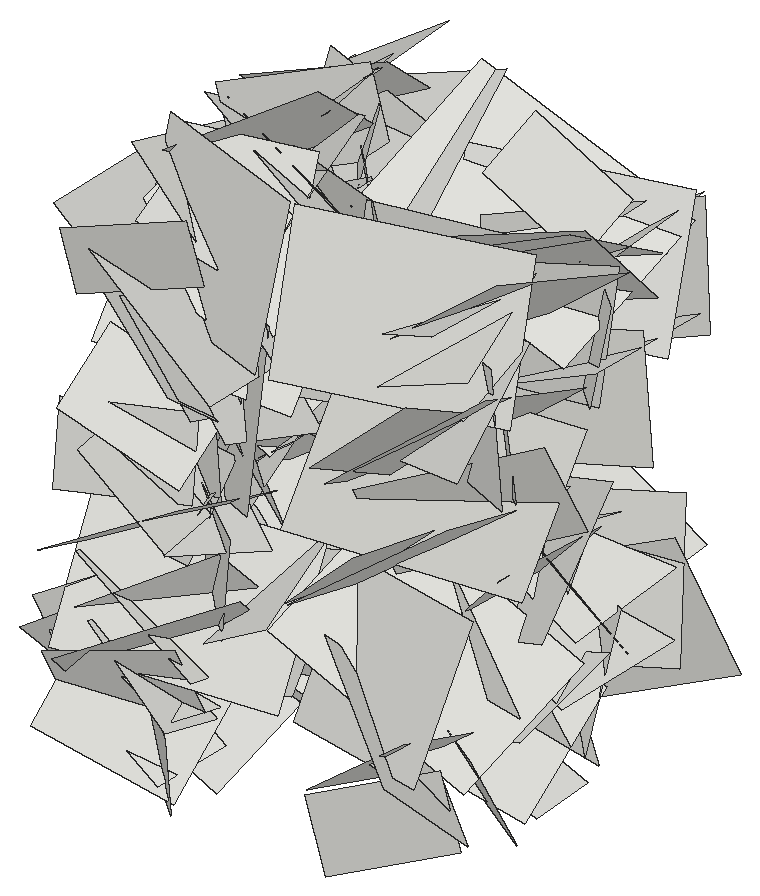
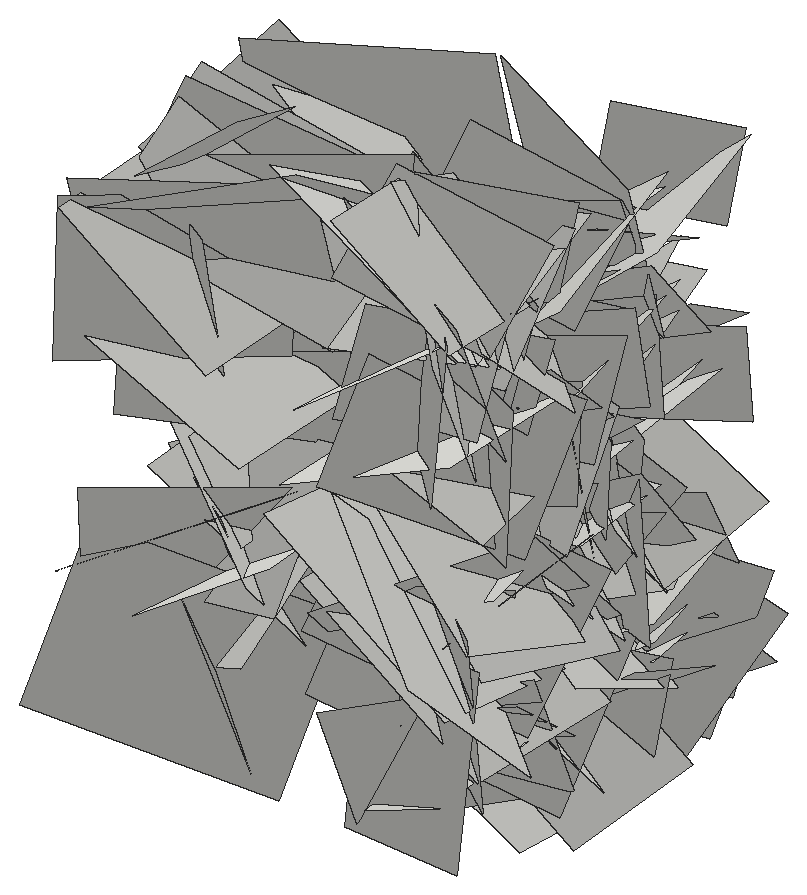
# SketchUp Ruby script. Lengths in inches.
U = 1.inch
M = Sketchup.active_model
def pt(a) = Geom::Point3d.new(a.map { |v| v * U })
def face(e, loops, mat)
  f = e.add_face(loops[0].map { |a| pt(a) })
  loops[1..].each { |l| e.add_face(l.map { |a| pt(a) }).erase! }
  f.material = f.back_material = mat if mat
  f
end
# faces: each face lists its corners as indices into pts; further lists are holes
def faces(e, pts, list, mat = nil) = list.each { |f| face(e, (f[0].is_a?(Array) ? f : [f]).map { |l| l.map { |i| pts[i] } }, mat) }
# xy, xz, yz: faces in a plane at the given z, y or x. An outline is a flat list of corners, or four numbers for a rectangle; further outlines are holes
def ring(l) = l.size == 4 ? [[l[0], l[1]], [l[2], l[1]], [l[2], l[3]], [l[0], l[3]]] : l.each_slice(2).to_a
def flat(e, list, mat, &to3) = list.each { |f| face(e, (f[0].is_a?(Array) ? f : [f]).map { |l| ring(l).map { |u, v| to3.(u, v) } }, mat) }
def xy(e, z, list, mat = nil) = flat(e, list, mat) { |x, y| [x, y, z] }
def xz(e, y, list, mat = nil) = flat(e, list, mat) { |x, z| [x, y, z] }
def yz(e, x, list, mat = nil) = flat(e, list, mat) { |y, z| [x, y, z] }
def lines(e, pts, list) = list.each { |a, b| e.add_line(pt(pts[a]), pt(pts[b])) }
# prism: a flat outline (further loops are holes) pulled along v
def prism(e, loops, v, mat = nil)
  f = face(e, loops, mat); d = Geom::Vector3d.new(v.map { |x| x * U })
  f.pushpull(f.normal.samedirection?(d) ? d.length : -d.length)
end
def box(e, o, s, mat = nil) = prism(e, [[o, [o[0] + s[0], o[1], o[2]], [o[0] + s[0], o[1] + s[1], o[2]], [o[0], o[1] + s[1], o[2]]]], [0, 0, s[2]], mat)
def at(x, y, z, deg = 0) = Geom::Transformation.translation(pt([x, y, z])) * Geom::Transformation.rotation(ORIGIN, Z_AXIS, deg.degrees)
def axes(o, x, y, z) = Geom::Transformation.new([*x, 0, *y, 0, *z, 0, *pt(o).to_a, 1])
def part(name) = M.definitions.add(name)
# library, detail: a bought-in or finely detailed component or shape, given as its bounding box
def library(name, o, s) = part(name).tap { |d| box(d.entities, o, s) }
def detail(e, o, s) = box(e.add_group.entities, o, s)
def put(e, d, t, mat = nil) = e.add_instance(d, t).tap { |i| i.material = mat if mat }
def group(e, t, mat = nil) = e.add_group.tap { |g| g.transformation = t; g.material = mat if mat }.entities
root = M.entities
c1 = part("Component\#6")
p = [[0.01,0,0],[0,3.24,4.54],[4.32,3.24,4.54],[4.33,0,0]]
faces(c1.entities,p,[[0,1,2,3]])
put(root,c1,axes([414.68,175.72,36.8],[0.15665,0.75943,0.7145],[0.11122,0.70715,-0.77331],[-1.09966,0.17971,0.02357]))
put(root,c1,axes([410.71,182.09,31.375],[0.0562,-0.72005,0.10613],[0.07977,0.11126,0.71729],[0.76737,0.04117,-0.08234]))
put(root,c1,axes([414.68,170.91,25.11],[-0.00896,0.33986,-0.6335],[-0.15678,-0.62081,-0.33108],[-0.74574,0.12644,0.07722]))
put(root,c1,axes([414.68,181.67,36.78],[0.05967,0.56874,-0.94691],[0.29528,-0.9248,-0.5389],[-1.13301,-0.21107,-0.19031]))
put(root,c1,axes([414.68,180.66,33.34],[0.08177,-0.45253,0.73357],[-0.03972,0.73405,0.45677],[-0.91278,-0.07248,0.04584]))
put(root,c1,axes([410.71,176.52,27.27],[0.06139,-0.83333,-0.30669],[-0.14477,-0.31205,0.82208],[0.93005,0.00643,0.1482]))
put(root,c1,axes([410.71,174.67,32.54],[-0.17055,0.3665,0.95024],[-0.03456,0.95968,-0.37566],[1.07902,0.08867,0.13816]))
put(root,c1,axes([410.71,177.99,23.55],[0.04107,0.5427,0.4395],[0.20397,0.41484,-0.52921],[0.71159,-0.15024,0.12632]))
put(root,c1,axes([410.71,177.89,30.77],[0.05678,-0.11721,0.8526],[-0.09083,0.84928,0.12214],[0.90772,0.09231,-0.04111]))
put(root,c1,axes([410.71,174.875,32.24],[0.12053,0.70886,0.38052],[-0.08644,0.39248,-0.70676],[0.84842,-0.06072,-0.12606]))
put(root,c1,axes([410.71,176.26,32.94],[0.03084,0.60524,0.59943],[-0.03406,0.60013,-0.60439],[0.90231,0.00196,-0.0433]))
put(root,c1,axes([410.71,169.05,21.98],[0.04882,0.58162,0.59704],[-0.02934,0.59868,-0.58109],[0.88303,-0.01226,-0.05232]))
put(root,c1,axes([410.71,171.18,26.98],[-0.09963,0.88743,-0.23237],[0.05305,-0.22828,-0.89204],[0.97094,0.10354,0.02489]))
put(root,c1,axes([410.71,174.16,29.86],[0.19319,0.59277,-0.26834],[0.07097,-0.29428,-0.60458],[0.68606,-0.13648,0.1381]))
put(root,c1,axes([414.68,171.52,27.71],[0.03995,0.48298,0.66079],[0.01207,0.66111,-0.48387],[-0.8675,0.03144,0.0237]))
put(root,c1,axes([410.71,174.95,31.63],[0.12097,-0.07785,-0.70642],[0.09105,-0.70871,0.09198],[0.74781,0.09888,0.10307]))
put(root,c1,axes([410.71,178.01,36.42],[0.04909,-0.68925,0.58112],[-0.09024,0.57594,0.68989],[0.95135,0.0902,0.03545]))
put(root,c1,axes([410.71,172,20.82],[-0.19013,-0.4174,1.11707],[-0.18593,1.12659,0.39279],[1.25031,0.10406,0.22828]))
put(root,c1,axes([414.68,172.01,32.68],[-0.01531,-0.04852,-0.71126],[-0.05574,-0.70939,0.04946],[-0.75363,0.05345,0.01079]))
put(root,c1,axes([410.71,184.3,37.98],[-0.01849,-0.42221,-1.00939],[-0.24573,-0.98518,0.41609],[1.13346,-0.22047,0.07374]))
put(root,c1,axes([410.71,183.5625,38.07],[0.03427,-0.86867,-0.02883],[-0.01016,-0.0292,0.8692],[0.92124,0.03199,0.01066]))
put(root,c1,axes([410.71,175.14,30.45],[-0.22771,0.17317,-1.07869],[0.0194,-1.09862,-0.18001],[1.15789,0.05246,-0.20912]))
put(root,c1,axes([414.68,173.36,27.66],[0.12062,0.63946,0.63128],[0.06443,0.62939,-0.6485],[-0.9503,0.12384,0.03616]))
put(root,c1,axes([414.68,173.29,20.87],[-0.09428,-0.62013,-0.08152],[-0.03551,-0.0775,0.6261],[-0.66205,0.09247,-0.02197]))
put(root,c1,axes([410.71,180.04,24.28],[0.15161,0.71603,-0.23582],[0.04269,-0.24694,-0.72538],[0.79796,-0.12284,0.08362]))
put(root,c1,axes([410.71,178.05,19.9375],[-0.14578,-1.0409,0.22357],[-0.02192,0.228,1.04879],[1.1283,-0.13006,0.04926]))
put(root,c1,axes([410.71,171.36,22.89],[0.02535,0.88672,0.32576],[-0.06435,0.32663,-0.88464],[0.99927,-0.00146,-0.06523]))
put(root,c1,axes([410.71,176.41,32.2],[0.11408,-0.0942,-0.79779],[0.0272,-0.8041,0.09841],[0.85109,0.03832,0.10379]))
put(root,c1,axes([414.68,177.7,39.03],[0.08239,-0.33737,-0.64844],[-0.10668,-0.65083,0.32654],[-0.76743,0.05425,-0.11501]))
put(root,c1,axes([410.71,181.8125,37.17],[-0.0246,-0.63961,0.56311],[0.17949,0.54862,0.63013],[0.88529,-0.129,-0.11211]))
put(root,c1,axes([410.71,173.5,20.5],[-0.29119,-0.77592,0.90535],[0.00734,0.92801,0.79744],[1.26387,-0.18415,0.20396]))
put(root,c1,axes([410.71,172.625,27.43],[-0.01975,0.58315,0.74345],[0.01761,0.74368,-0.58292],[1.00141,-0.00157,0.02491]))
put(root,c1,axes([410.71,172.13,35.78],[0.07615,0.65901,-0.5201],[0.04859,-0.52431,-0.658],[0.88857,-0.02781,0.08055]))
put(root,c1,axes([410.71,177.13,31.79],[-0.078,-0.30439,1.03044],[-0.07955,1.03178,0.29943],[1.13614,0.05135,0.09171]))
put(root,c1,axes([410.71,182.1,27.04],[-0.18817,-1.1788,-0.21223],[-0.10509,-0.19936,1.19019],[1.26526,-0.19187,0.06729]))
put(root,c1,axes([414.68,180.11,41],[0.0874,0.13713,-0.78202],[0.02965,-0.78624,-0.13492],[-0.84107,-0.01347,-0.08602]))
put(root,c1,axes([414.68,171.42,39.46],[-0.01769,0.21401,-0.61924],[-0.03571,-0.6189,-0.21298],[-0.69357,0.02641,0.02676]))
put(root,c1,axes([414.68,174.375,32.02],[0.18574,0.64681,-0.5499],[0.00393,-0.56207,-0.65994],[-0.8999,0.13105,-0.11638]))
put(root,c1,axes([414.68,173.15,22.23],[-0.01199,-0.5915,0.12784],[-0.10227,0.12799,0.58366],[-0.63327,-0.00947,-0.09668]))
put(root,c1,axes([410.71,170.16,39.2],[-0.24703,1.2789,-0.21613],[-0.13589,-0.24123,-1.28918],[1.36812,0.20696,-0.16707]))
put(root,c1,axes([410.71,174.01,26.46],[-0.07872,-0.97306,0.24072],[0.0738,0.23579,0.97461],[1.05998,-0.08868,-0.04998]))
put(root,c1,axes([414.68,173.67,32.24],[0.05341,-0.65994,-0.37026],[0.06447,-0.36634,0.66124],[-0.79951,-0.07362,0.02859]))
put(root,c1,axes([414.68,175.43,34.87],[0.0411,0.62613,0.35799],[0.03637,0.3565,-0.62724],[-0.76365,0.05068,-0.01061]))
put(root,c1,axes([410.71,185.38,28.27],[-0.28552,-0.8956,-0.93898],[-0.07116,-0.9481,0.92355],[1.37362,-0.23528,-0.14733]))
put(root,c1,axes([410.71,182.77,28.15],[-0.11013,-1.0722,-0.31704],[-0.03816,-0.31503,1.07721],[1.18456,-0.10983,0.00522]))
put(root,c1,axes([410.71,176.05,33.17],[0.01986,0.50916,-0.88553],[-0.06176,-0.8837,-0.50934],[1.08099,-0.05984,-0.01283]))
put(root,c1,axes([414.68,182.27,37.76],[0.22679,0.05489,-0.89691],[0.06736,-0.9206,-0.04118],[-0.95012,-0.05216,-0.217]))
put(root,c1,axes([410.71,174.9,23.69],[-0.06803,0.90477,0.33383],[0.16872,0.33992,-0.89067],[1.00823,0.00417,0.17157]))
put(root,c1,axes([414.68,173.11,21.9],[0.05319,-0.68826,0.19248],[0.04456,0.19546,0.68797],[-0.75624,-0.03689,0.05408]))
put(root,c1,axes([414.68,178.15,33.23],[-0.08938,-0.00525,-0.60269],[0.06829,-0.60515,-0.00374],[-0.63521,-0.06432,0.0844]))
put(root,c1,axes([414.68,176.44,21.6],[0.04345,0.60879,-0.00304],[-0.10651,0.00376,-0.60183],[-0.63647,0.04093,0.10051]))
put(root,c1,axes([410.71,183.67,38.38],[0.04708,0.10578,-1.15378],[-0.2342,-1.13267,-0.11235],[1.2056,-0.22416,0.02323]))
put(root,c1,axes([410.71,173.31,35.98],[-0.01252,1.07454,-0.37217],[-0.12805,-0.37127,-1.06811],[1.19858,-0.02844,-0.11799]))
put(root,c1,axes([410.71,174.78,20.26],[0.10048,-0.39109,0.79293],[0.10042,0.79738,0.38196],[0.93179,-0.04376,-0.12667]))
put(root,c1,axes([414.68,180.68,27.18],[0.06604,-0.60003,0.10008],[-0.10227,0.08959,0.59716],[-0.63666,-0.07663,-0.08554]))
put(root,c1,axes([414.68,170.73,19.61],[0.06378,-0.15247,0.68566],[0.07422,0.68605,0.14641],[-0.74085,0.05561,0.0737]))
put(root,c1,axes([410.71,178.01,21.81],[0.00864,0.40014,0.99077],[-0.02339,0.99065,-0.39991],[1.13239,0.01741,-0.01582]))
put(root,c1,axes([414.68,178.13,40.15],[0.04908,0.64392,0.19174],[0.08573,0.18545,-0.64234],[-0.70699,0.06719,-0.06458]))
put(root,c1,axes([410.71,171.95,33.74],[-0.07102,0.70639,0.8167],[0.11892,0.8184,-0.69866],[1.13841,-0.04142,0.12393]))
put(root,c1,axes([414.68,176.07,37.03],[0.15674,-0.62528,-0.09698],[-0.10666,-0.12156,0.63036],[-0.66219,-0.12843,-0.12449]))
put(root,c1,axes([414.68,180.42,25.12],[0.17902,-0.88337,-0.09354],[0.21931,-0.05348,0.8786],[-0.91571,-0.1855,0.19214]))
put(root,c1,axes([410.71,172.46,21.25],[0.14489,-0.73421,0.72244],[-0.08794,0.71856,0.74596],[1.0883,0.15581,-0.0359]))
put(root,c1,axes([410.71,171.47,32.36],[0.16942,0.96147,-0.31887],[-0.08969,-0.30901,-0.97416],[1.06999,-0.17814,-0.03117]))
put(root,c1,axes([410.71,179.35,38.14],[0.07028,1.07405,0.02302],[-0.04111,0.02544,-1.07534],[1.13802,-0.06541,-0.04027]))
put(root,c1,axes([414.68,181.39,28.46],[0.11732,-0.15238,-0.58962],[-0.01785,-0.59981,0.15186],[-0.64528,-0.01111,-0.1114]))
put(root,c1,axes([414.68,173.74,31.89],[0.15856,-0.67469,0.29232],[0.1064,0.31425,0.67394],[-0.77211,-0.09525,0.1529]))
put(root,c1,axes([410.71,173.84,39.64],[-0.13369,1.27699,-0.41872],[-0.11509,-0.42887,-1.27523],[1.41986,0.08547,-0.14279]))
put(root,c1,axes([414.68,172.58,29],[0.14706,-0.68518,0.03236],[0.10474,0.05263,0.69082],[-0.71951,-0.13238,0.10718]))
put(root,c1,axes([410.71,180.75,35.09],[-0.01445,0.08276,-1.11066],[0.1396,-1.10283,-0.0838],[1.17228,0.13235,-0.00371]))
put(root,c1,axes([410.71,182.25,27.43],[-0.1955,0.46825,-1.21407],[0.10064,-1.21809,-0.48422],[1.37564,0.15566,-0.13711]))
put(root,c1,axes([410.71,175.96,26.52],[0.03553,0.82214,0.9074],[-0.07429,0.90754,-0.81968],[1.2958,0.02948,-0.07187]))
put(root,c1,axes([410.71,172.47,36.95],[0.1233,0.89549,0.4145],[0.21728,0.38634,-0.89217],[1.02316,-0.18996,0.13951]))
put(root,c1,axes([410.71,183.25,38.77],[-0.07927,-0.40868,-1.12281],[0.1988,-1.11508,0.39337],[1.25087,0.15132,-0.13368]))
put(root,c1,axes([410.71,179.04,23.77],[0.11323,-0.75693,-0.7774],[0.09292,-0.77258,0.76428],[1.14637,0.13739,0.01483]))
put(root,c1,axes([410.71,182.77,28.7],[-0.0358,-0.11408,-1.31406],[-0.04325,-1.31377,0.1151],[1.39747,-0.04358,-0.0301]))
put(root,c1,axes([410.71,180.07,24.39],[-0.06666,-0.76105,0.92501],[0.21989,0.90537,0.75899],[1.25053,-0.19976,-0.08415]))
put(root,c1,axes([410.71,177.97,39.67],[-0.02985,0.75948,-0.84861],[0.27983,-0.8214,-0.74388],[1.17429,0.21504,0.15569]))
put(root,c1,axes([410.71,174.06,31.875],[0.08593,-0.00736,1.08266],[0.18405,1.07173,-0.00571],[1.1328,-0.17357,-0.0812]))
put(root,c1,axes([410.71,182.31,23.94],[-0.04872,-1.30982,0.04089],[0.01644,0.04037,1.31055],[1.38898,-0.04642,-0.01408]))
put(root,c1,axes([410.71,178.49,34.59],[0.00763,1.14917,-0.03145],[0.21412,-0.03223,-1.13128],[1.19962,-0.00155,0.20212]))
put(root,c1,axes([410.71,178.09,32.9],[0.18757,-0.47698,-1.21124],[-0.23196,-1.21588,0.44684],[1.36024,-0.14157,0.24323]))
put(root,c1,axes([410.71,178.68,21.25],[0.14964,-1.02559,0.91665],[-0.24358,0.89093,1.03221],[1.43757,0.25771,0.07948]))
put(root,c1,axes([410.71,169.91,24.28],[-0.0494,0.58776,1.07494],[0.25393,1.05932,-0.56884],[1.27358,-0.18841,0.15511]))
put(root,c1,axes([410.71,175.66,39.88],[-0.03914,-0.32872,-1.22009],[0.25418,-1.20026,0.31612],[1.31508,0.2222,-0.09741]))
put(root,c1,axes([410.71,177.96,25.04],[0.10915,-1.1796,-0.55067],[0.03689,-0.5497,1.18402],[1.37942,0.10803,0.01191]))
put(root,c1,axes([410.71,183.77,26.5],[0.0762,-1.33255,-0.21023],[0.04546,-0.20817,1.33413],[1.42926,0.07766,-0.03122]))
put(root,c1,axes([410.71,177.28,39.83],[0.04784,1.11638,-0.64936],[0.22797,-0.64718,-1.09769],[1.34988,0.06974,0.20839]))
put(root,c1,axes([410.71,179.625,37.91],[0.28026,0.12179,-1.29213],[0.26115,-1.29941,-0.07206],[1.35072,0.22596,0.28204]))
put(root,c1,axes([410.71,183.19,37.72],[0.19709,-1.17807,-0.70591],[0.26547,-0.67132,1.18631],[1.43137,0.28672,-0.12282]))
put(root,c1,axes([424.49,183.19,37.72],[-0.19709,-1.17807,-0.70591],[-0.26547,-0.67132,1.18631],[-1.43137,0.28672,-0.12282]))
put(root,c1,axes([424.49,179.625,37.91],[-0.28026,0.12179,-1.29213],[-0.26115,-1.29941,-0.07206],[-1.35072,0.22596,0.28204]))
put(root,c1,axes([424.49,177.28,39.83],[-0.04784,1.11638,-0.64936],[-0.22797,-0.64718,-1.09769],[-1.34988,0.06974,0.20839]))
put(root,c1,axes([424.49,183.77,26.5],[-0.0762,-1.33255,-0.21023],[-0.04546,-0.20817,1.33413],[-1.42926,0.07766,-0.03122]))
put(root,c1,axes([424.49,177.96,25.04],[-0.10915,-1.1796,-0.55067],[-0.03689,-0.5497,1.18402],[-1.37942,0.10803,0.01191]))
put(root,c1,axes([424.49,175.66,39.88],[0.03914,-0.32872,-1.22009],[-0.25418,-1.20026,0.31612],[-1.31508,0.2222,-0.09741]))
put(root,c1,axes([424.49,169.91,24.28],[0.0494,0.58776,1.07494],[-0.25393,1.05932,-0.56884],[-1.27358,-0.18841,0.15511]))
put(root,c1,axes([424.49,178.68,21.25],[-0.14964,-1.02559,0.91665],[0.24358,0.89093,1.03221],[-1.43757,0.25771,0.07948]))
put(root,c1,axes([424.49,178.09,32.9],[-0.18757,-0.47698,-1.21124],[0.23196,-1.21588,0.44684],[-1.36024,-0.14157,0.24323]))
put(root,c1,axes([424.49,178.49,34.59],[-0.00763,1.14917,-0.03145],[-0.21412,-0.03223,-1.13128],[-1.19962,-0.00155,0.20212]))
put(root,c1,axes([424.49,182.31,23.94],[0.04872,-1.30982,0.04089],[-0.01644,0.04037,1.31055],[-1.38898,-0.04642,-0.01408]))
put(root,c1,axes([424.49,174.06,31.875],[-0.08593,-0.00736,1.08266],[-0.18405,1.07173,-0.00571],[-1.1328,-0.17357,-0.0812]))
put(root,c1,axes([424.49,177.97,39.67],[0.02985,0.75948,-0.84861],[-0.27983,-0.8214,-0.74388],[-1.17429,0.21504,0.15569]))
put(root,c1,axes([424.49,180.07,24.39],[0.06666,-0.76105,0.92501],[-0.21989,0.90537,0.75899],[-1.25053,-0.19976,-0.08415]))
put(root,c1,axes([424.49,182.77,28.7],[0.0358,-0.11408,-1.31406],[0.04325,-1.31377,0.1151],[-1.39747,-0.04358,-0.0301]))
put(root,c1,axes([424.49,179.04,23.77],[-0.11323,-0.75693,-0.7774],[-0.09292,-0.77258,0.76428],[-1.14637,0.13739,0.01483]))
put(root,c1,axes([424.49,183.25,38.77],[0.07927,-0.40868,-1.12281],[-0.1988,-1.11508,0.39337],[-1.25087,0.15132,-0.13368]))
put(root,c1,axes([424.49,172.47,36.95],[-0.1233,0.89549,0.4145],[-0.21728,0.38634,-0.89217],[-1.02316,-0.18996,0.13951]))
put(root,c1,axes([424.49,175.96,26.52],[-0.03553,0.82214,0.9074],[0.07429,0.90754,-0.81968],[-1.2958,0.02948,-0.07187]))
put(root,c1,axes([424.49,182.25,27.43],[0.1955,0.46825,-1.21407],[-0.10064,-1.21809,-0.48422],[-1.37564,0.15566,-0.13711]))
put(root,c1,axes([424.49,180.75,35.09],[0.01445,0.08276,-1.11066],[-0.1396,-1.10283,-0.0838],[-1.17228,0.13235,-0.00371]))
put(root,c1,axes([420.52,172.58,29],[-0.14706,-0.68518,0.03236],[-0.10474,0.05263,0.69082],[0.71951,-0.13238,0.10718]))
put(root,c1,axes([424.49,173.84,39.64],[0.13369,1.27699,-0.41872],[0.11509,-0.42887,-1.27523],[-1.41986,0.08547,-0.14279]))
put(root,c1,axes([420.52,173.74,31.89],[-0.15856,-0.67469,0.29232],[-0.1064,0.31425,0.67394],[0.77211,-0.09525,0.1529]))
put(root,c1,axes([420.52,181.39,28.46],[-0.11732,-0.15238,-0.58962],[0.01785,-0.59981,0.15186],[0.64528,-0.01111,-0.1114]))
put(root,c1,axes([424.49,179.35,38.14],[-0.07028,1.07405,0.02302],[0.04111,0.02544,-1.07534],[-1.13802,-0.06541,-0.04027]))
put(root,c1,axes([424.49,171.47,32.36],[-0.16942,0.96147,-0.31887],[0.08969,-0.30901,-0.97416],[-1.06999,-0.17814,-0.03117]))
put(root,c1,axes([424.49,172.46,21.25],[-0.14489,-0.73421,0.72244],[0.08794,0.71856,0.74596],[-1.0883,0.15581,-0.0359]))
put(root,c1,axes([420.52,180.42,25.12],[-0.17902,-0.88337,-0.09354],[-0.21931,-0.05348,0.8786],[0.91571,-0.1855,0.19214]))
put(root,c1,axes([420.52,176.07,37.03],[-0.15674,-0.62528,-0.09698],[0.10666,-0.12156,0.63036],[0.66219,-0.12843,-0.12449]))
put(root,c1,axes([424.49,171.95,33.74],[0.07102,0.70639,0.8167],[-0.11892,0.8184,-0.69866],[-1.13841,-0.04142,0.12393]))
put(root,c1,axes([420.52,178.13,40.15],[-0.04908,0.64392,0.19174],[-0.08573,0.18545,-0.64234],[0.70699,0.06719,-0.06458]))
put(root,c1,axes([424.49,178.01,21.81],[-0.00864,0.40014,0.99077],[0.02339,0.99065,-0.39991],[-1.13239,0.01741,-0.01582]))
put(root,c1,axes([420.52,170.73,19.61],[-0.06378,-0.15247,0.68566],[-0.07422,0.68605,0.14641],[0.74085,0.05561,0.0737]))
put(root,c1,axes([420.52,180.68,27.18],[-0.06604,-0.60003,0.10008],[0.10227,0.08959,0.59716],[0.63666,-0.07663,-0.08554]))
put(root,c1,axes([424.49,174.78,20.26],[-0.10048,-0.39109,0.79293],[-0.10042,0.79738,0.38196],[-0.93179,-0.04376,-0.12667]))
put(root,c1,axes([424.49,173.31,35.98],[0.01252,1.07454,-0.37217],[0.12805,-0.37127,-1.06811],[-1.19858,-0.02844,-0.11799]))
put(root,c1,axes([424.49,183.67,38.38],[-0.04708,0.10578,-1.15378],[0.2342,-1.13267,-0.11235],[-1.2056,-0.22416,0.02323]))
put(root,c1,axes([420.52,176.44,21.6],[-0.04345,0.60879,-0.00304],[0.10651,0.00376,-0.60183],[0.63647,0.04093,0.10051]))
put(root,c1,axes([420.52,178.15,33.23],[0.08938,-0.00525,-0.60269],[-0.06829,-0.60515,-0.00374],[0.63521,-0.06432,0.0844]))
put(root,c1,axes([420.52,173.11,21.9],[-0.05319,-0.68826,0.19248],[-0.04456,0.19546,0.68797],[0.75624,-0.03689,0.05408]))
put(root,c1,axes([424.49,174.9,23.69],[0.06803,0.90477,0.33383],[-0.16872,0.33992,-0.89067],[-1.00823,0.00417,0.17157]))
put(root,c1,axes([420.52,182.27,37.76],[-0.22679,0.05489,-0.89691],[-0.06736,-0.9206,-0.04118],[0.95012,-0.05216,-0.217]))
put(root,c1,axes([424.49,176.05,33.17],[-0.01986,0.50916,-0.88553],[0.06176,-0.8837,-0.50934],[-1.08099,-0.05984,-0.01283]))
